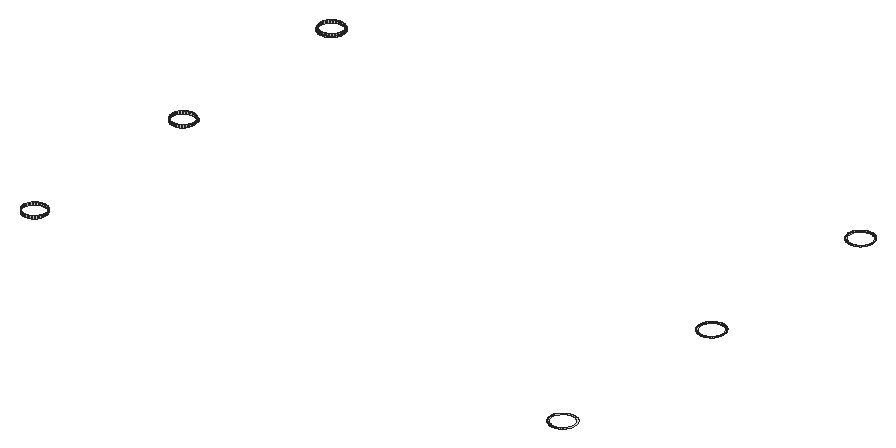
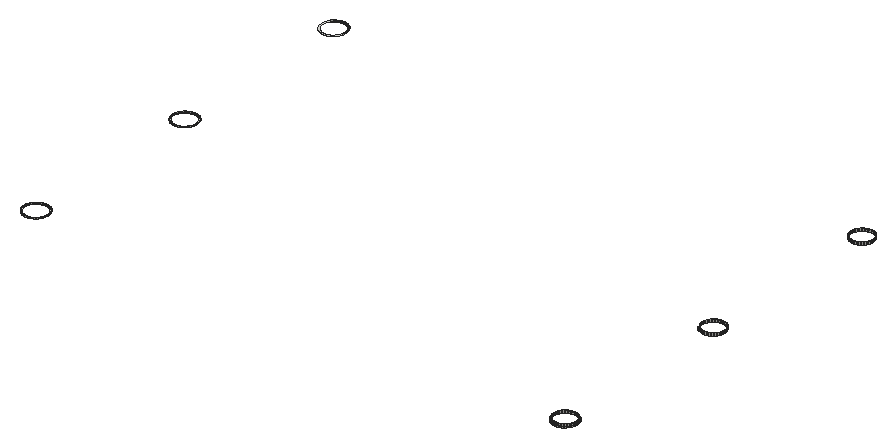
# SketchUp Ruby script. Lengths in inches.
U = 1.inch
M = Sketchup.active_model
def pt(a) = Geom::Point3d.new(a.map { |v| v * U })
def face(e, loops, mat)
  f = e.add_face(loops[0].map { |a| pt(a) })
  loops[1..].each { |l| e.add_face(l.map { |a| pt(a) }).erase! }
  f.material = f.back_material = mat if mat
  f
end
# faces: each face lists its corners as indices into pts; further lists are holes
def faces(e, pts, list, mat = nil) = list.each { |f| face(e, (f[0].is_a?(Array) ? f : [f]).map { |l| l.map { |i| pts[i] } }, mat) }
# xy, xz, yz: faces in a plane at the given z, y or x. An outline is a flat list of corners, or four numbers for a rectangle; further outlines are holes
def ring(l) = l.size == 4 ? [[l[0], l[1]], [l[2], l[1]], [l[2], l[3]], [l[0], l[3]]] : l.each_slice(2).to_a
def flat(e, list, mat, &to3) = list.each { |f| face(e, (f[0].is_a?(Array) ? f : [f]).map { |l| ring(l).map { |u, v| to3.(u, v) } }, mat) }
def xy(e, z, list, mat = nil) = flat(e, list, mat) { |x, y| [x, y, z] }
def xz(e, y, list, mat = nil) = flat(e, list, mat) { |x, z| [x, y, z] }
def yz(e, x, list, mat = nil) = flat(e, list, mat) { |y, z| [x, y, z] }
def lines(e, pts, list) = list.each { |a, b| e.add_line(pt(pts[a]), pt(pts[b])) }
# prism: a flat outline (further loops are holes) pulled along v
def prism(e, loops, v, mat = nil)
  f = face(e, loops, mat); d = Geom::Vector3d.new(v.map { |x| x * U })
  f.pushpull(f.normal.samedirection?(d) ? d.length : -d.length)
end
def box(e, o, s, mat = nil) = prism(e, [[o, [o[0] + s[0], o[1], o[2]], [o[0] + s[0], o[1] + s[1], o[2]], [o[0], o[1] + s[1], o[2]]]], [0, 0, s[2]], mat)
def at(x, y, z, deg = 0) = Geom::Transformation.translation(pt([x, y, z])) * Geom::Transformation.rotation(ORIGIN, Z_AXIS, deg.degrees)
def axes(o, x, y, z) = Geom::Transformation.new([*x, 0, *y, 0, *z, 0, *pt(o).to_a, 1])
def part(name) = M.definitions.add(name)
# library, detail: a bought-in or finely detailed component or shape, given as its bounding box
def library(name, o, s) = part(name).tap { |d| box(d.entities, o, s) }
def detail(e, o, s) = box(e.add_group.entities, o, s)
def put(e, d, t, mat = nil) = e.add_instance(d, t).tap { |i| i.material = mat if mat }
def group(e, t, mat = nil) = e.add_group.tap { |g| g.transformation = t; g.material = mat if mat }.entities
root = M.entities
xy(root,113.9,[[[112.03,39.21,111.8,39.22,111.57,39.26,111.35,39.3125,111.13,39.39,110.92,39.5,110.73,39.62,110.55,39.76,110.38,39.92,110.24,40.1,110.11,40.29,110,40.49,109.92,40.71,109.85,40.93,109.82,41.16,109.8,41.39,109.81,41.62,109.84,41.85,109.9,42.07,109.98,42.28,110.08,42.49,110.2,42.69,110.35,42.87,110.51,43.03,110.69,43.18,110.875,43.31,111.08,43.41,111.29,43.5,111.52,43.56,111.74,43.6,111.97,43.61,112.2,43.6,112.43,43.57,112.65,43.51,112.87,43.43,113.08,43.33,113.27,43.21,113.45,43.07,113.62,42.91,113.76,42.73,113.89,42.54,114,42.33,114.08,42.12,114.15,41.9,114.18,41.67,114.2,41.44,114.19,41.21,114.16,40.98,114.1,40.76,114.02,40.54,113.92,40.34,113.8,40.14,113.65,39.96,113.49,39.8,113.31,39.65,113.125,39.52,112.92,39.42,112.71,39.33,112.48,39.27,112.26,39.23],[112.02,39.41,112.23,39.43,112.44,39.46,112.64,39.52,112.84,39.6,113.02,39.69,113.2,39.8125,113.36,39.94,113.5,40.09,113.63,40.26,113.74,40.44,113.84,40.625,113.91,40.82,113.96,41.02,113.99,41.23,114,41.4375,113.99,41.65,113.95,41.85,113.89,42.06,113.82,42.25,113.72,42.44,113.6,42.61,113.47,42.77,113.32,42.92,113.16,43.05,112.98,43.16,112.79,43.25,112.59,43.32,112.39,43.375,112.18,43.41,111.98,43.41,111.77,43.4,111.56,43.37,111.36,43.31,111.16,43.23,110.98,43.13,110.8,43.02,110.64,42.88,110.5,42.73,110.37,42.57,110.26,42.39,110.16,42.21,110.09,42.01,110.04,41.81,110.01,41.6,110,41.39,110.01,41.18,110.05,40.97,110.11,40.77,110.18,40.58,110.28,40.39,110.4,40.22,110.53,40.06,110.68,39.91,110.84,39.78,111.02,39.67,111.21,39.58,111.41,39.5,111.61,39.45,111.82,39.42]],[[112.03,72.63,111.8,72.64,111.57,72.67,111.35,72.73,111.13,72.81,110.92,72.91,110.73,73.03,110.55,73.18,110.38,73.34,110.24,73.51,110.11,73.7,110,73.91,109.92,74.12,109.85,74.34,109.82,74.57,109.8,74.8,109.81,75.03,109.84,75.26,109.9,75.48,109.98,75.7,110.08,75.9,110.2,76.1,110.35,76.28,110.51,76.44,110.69,76.59,110.875,76.72,111.08,76.83,111.29,76.91,111.52,76.97,111.74,77.01,111.97,77.03,112.2,77.02,112.43,76.99,112.65,76.93,112.87,76.85,113.08,76.75,113.27,76.625,113.45,76.48,113.62,76.32,113.76,76.14,113.89,75.95,114,75.75,114.08,75.53,114.15,75.3125,114.18,75.08,114.2,74.86,114.19,74.625,114.16,74.4,114.1,74.17,114.02,73.96,113.92,73.75,113.8,73.56,113.65,73.375,113.49,73.21,113.31,73.0625,113.125,72.9375,112.92,72.83,112.71,72.74,112.48,72.68,112.26,72.64],[112.02,72.83,112.23,72.84,112.44,72.88,112.64,72.93,112.84,73.01,113.02,73.11,113.2,73.22,113.36,73.36,113.5,73.51,113.63,73.67,113.74,73.85,113.84,74.04,113.91,74.23,113.96,74.4375,113.99,74.64,114,74.85,113.99,75.0625,113.95,75.27,113.89,75.47,113.82,75.66,113.72,75.85,113.6,76.02,113.47,76.18,113.32,76.33,113.16,76.46,112.98,76.57,112.79,76.67,112.59,76.74,112.39,76.79,112.18,76.82,111.98,76.83,111.77,76.8125,111.56,76.78,111.36,76.72,111.16,76.65,110.98,76.55,110.8,76.43,110.64,76.3,110.5,76.15,110.37,75.98,110.26,75.81,110.16,75.62,110.09,75.42,110.04,75.22,110.01,75.01,110,74.8,110.01,74.59,110.05,74.39,110.11,74.1875,110.18,73.99,110.28,73.81,110.4,73.63,110.53,73.47,110.68,73.33,110.84,73.2,111.02,73.08,111.21,72.99,111.41,72.92,111.61,72.87,111.82,72.84]],[[112.03,106.04,111.8,106.05,111.57,106.08,111.35,106.14,111.13,106.22,110.92,106.32,110.73,106.45,110.55,106.59,110.38,106.75,110.24,106.93,110.11,107.12,110,107.32,109.92,107.54,109.85,107.76,109.82,107.99,109.8,108.22,109.81,108.45,109.84,108.67,109.9,108.9,109.98,109.11,110.08,109.32,110.2,109.51,110.35,109.69,110.51,109.86,110.69,110.01,110.875,110.13,111.08,110.24,111.29,110.33,111.52,110.39,111.74,110.43,111.97,110.44,112.2,110.43,112.43,110.4,112.65,110.34,112.87,110.26,113.08,110.16,113.27,110.04,113.45,109.9,113.62,109.73,113.76,109.56,113.89,109.37,114,109.16,114.08,108.95,114.15,108.73,114.18,108.5,114.2,108.27,114.19,108.04,114.16,107.8125,114.1,107.59,114.02,107.37,113.92,107.17,113.8,106.97,113.65,106.79,113.49,106.625,113.31,106.48,113.125,106.35,112.92,106.24,112.71,106.16,112.48,106.1,112.26,106.06],[112.02,106.24,112.23,106.26,112.44,106.29,112.64,106.35,112.84,106.43,113.02,106.52,113.2,106.64,113.36,106.77,113.5,106.92,113.63,107.09,113.74,107.26,113.84,107.45,113.91,107.65,113.96,107.85,113.99,108.06,114,108.27,113.99,108.48,113.95,108.68,113.89,108.88,113.82,109.08,113.72,109.26,113.6,109.4375,113.47,109.6,113.32,109.74,113.16,109.875,112.98,109.99,112.79,110.08,112.59,110.15,112.39,110.2,112.18,110.23,111.98,110.24,111.77,110.23,111.56,110.19,111.36,110.14,111.16,110.06,110.98,109.96,110.8,109.85,110.64,109.71,110.5,109.5625,110.37,109.4,110.26,109.22,110.16,109.03,110.09,108.84,110.04,108.63,110.01,108.43,110,108.22,110.01,108.01,110.05,107.8,110.11,107.6,110.18,107.41,110.28,107.22,110.4,107.05,110.53,106.89,110.68,106.74,110.84,106.61,111.02,106.5,111.21,106.41,111.41,106.33,111.61,106.28,111.82,106.25]],[[16.81,106.41,16.58,106.42,16.35,106.44,16.125,106.49,15.91,106.5625,15.7,106.66,15.5,106.77,15.31,106.91,15.14,107.0625,14.99,107.23,14.86,107.42,14.74,107.62,14.65,107.83,14.58,108.05,14.54,108.27,14.51,108.5,14.52,108.73,14.54,108.96,14.59,109.18,14.66,109.4,14.76,109.61,14.87,109.81,15.01,109.99,15.16,110.16,15.33,110.32,15.52,110.45,15.72,110.5625,15.93,110.66,16.15,110.73,16.375,110.77,16.6,110.8,16.83,110.79,17.06,110.77,17.28,110.72,17.5,110.65,17.71,110.55,17.91,110.4375,18.09,110.3,18.26,110.15,18.42,109.97,18.55,109.79,18.66,109.59,18.76,109.38,18.83,109.16,18.87,108.94,18.89,108.71,18.89,108.48,18.87,108.25,18.82,108.02,18.75,107.81,18.65,107.6,18.54,107.4,18.4,107.21,18.25,107.05,18.07,106.89,17.89,106.76,17.6875,106.65,17.48,106.55,17.26,106.48,17.03,106.4375],[16.8,106.61,17,106.63,17.21,106.68,17.41,106.74,17.6,106.82,17.78,106.93,17.95,107.05,18.11,107.1875,18.25,107.34,18.37,107.51,18.47,107.69,18.5625,107.88,18.625,108.08,18.67,108.28,18.69,108.49,18.7,108.7,18.67,108.9,18.63,109.11,18.57,109.31,18.49,109.5,18.38,109.68,18.26,109.85,18.12,110.01,17.97,110.15,17.8,110.27,17.62,110.375,17.43,110.46,17.23,110.53,17.03,110.57,16.82,110.59,16.61,110.6,16.4,110.57,16.2,110.53,16,110.47,15.81,110.39,15.63,110.28,15.46,110.16,15.3,110.02,15.16,109.87,15.04,109.7,14.93,109.52,14.85,109.33,14.78,109.13,14.74,108.93,14.72,108.72,14.71,108.51,14.73,108.3,14.78,108.1,14.84,107.9,14.92,107.71,15.03,107.53,15.15,107.36,15.29,107.2,15.44,107.0625,15.61,106.94,15.79,106.83,15.98,106.75,16.18,106.68,16.38,106.64,16.59,106.62]]])
xz(root,39.92,[[16.59,113.9,16.8,114.33]])
xz(root,43.9,[[16.61,113.9,16.82,114.33]])
xz(root,73.27,[[16.59,113.9,16.8,114.34]])
xz(root,77.25,[[16.61,113.9,16.82,114.34]])
yz(root,18.89,[[108.48,113.9,108.71,114]])
p = [[111.8,39.22,114],[111.57,39.26,114],[111.57,39.26,113.9],[111.8,39.22,113.9],[112.03,39.21,114],[112.03,39.21,113.9],
  [112.26,39.23,114],[112.26,39.23,113.9],[112.48,39.27,114],[112.48,39.27,113.9],[111.35,39.3125,114],[111.13,39.39,114],
  [111.13,39.39,113.9],[111.35,39.3125,113.9],[112.71,39.33,114],[112.71,39.33,113.9],[112.92,39.42,114],[112.92,39.42,113.9],
  [110.92,39.5,114],[110.92,39.5,113.9],[113.125,39.52,114],[113.125,39.52,113.9],[110.73,39.62,114],[110.73,39.62,113.9],
  [113.31,39.65,114],[113.31,39.65,113.9],[110.55,39.76,114],[110.55,39.76,113.9],[113.49,39.8,114],[113.49,39.8,113.9],
  [110.38,39.92,114],[110.38,39.92,113.9],[113.65,39.96,114],[113.65,39.96,113.9],[16.38,39.94,113.9],[16.18,39.99,113.9],
  [16.18,39.99,114.33],[16.38,39.94,114.33],[16.59,39.92,113.9],[16.59,39.92,114.33],[17,39.94,113.9],[16.8,39.92,113.9],
  [16.8,39.92,114.33],[17,39.94,114.33],[17.21,39.98,113.9],[17.21,39.98,114.33],[110.24,40.1,114],[110.24,40.1,113.9],
  [15.98,40.05,113.9],[15.98,40.05,114.33],[17.41,40.05,113.9],[17.41,40.05,114.33],[17.6,40.13,113.9],[17.6,40.13,114.33],
  [15.79,40.14,113.9],[15.61,40.25,113.9],[15.61,40.25,114.33],[15.79,40.14,114.33],[17.78,40.23,113.9],[17.78,40.23,114.33],
  [110.11,40.29,114],[110.11,40.29,113.9],[15.44,40.37,113.9],[15.44,40.37,114.33],[17.95,40.35,113.9],[17.95,40.35,114.33],
  [110,40.49,114],[110,40.49,113.9],[15.29,40.51,113.9],[15.29,40.51,114.33],[18.11,40.49,113.9],[18.11,40.49,114.33],
  [15.15,40.67,113.9],[15.15,40.67,114.33],[18.25,40.65,113.9],[18.25,40.65,114.33],[109.92,40.71,114],[109.92,40.71,113.9],
  [18.37,40.82,113.9],[18.37,40.82,114.33],[15.03,40.84,113.9],[15.03,40.84,114.33],[109.85,40.93,114],[109.85,40.93,113.9],
  [14.92,41.02,113.9],[14.92,41.02,114.33],[18.47,41,113.9],[18.47,41,114.33],[109.82,41.16,114],[109.82,41.16,113.9],
  [14.84,41.21,113.9],[14.84,41.21,114.33],[18.5625,41.1875,113.9],[18.5625,41.1875,114.33],[14.78,41.41,113.9],[14.78,41.41,114.33],
  [18.625,41.38,113.9],[18.625,41.38,114.33],[109.8,41.39,114],[109.8,41.39,113.9],[14.73,41.61,113.9],[14.73,41.61,114.33],
  [18.67,41.59,113.9],[18.67,41.59,114.33],[109.81,41.62,114],[109.81,41.62,113.9],[14.71,41.82,113.9],[14.71,41.82,114.33],
  [18.69,41.79,113.9],[18.69,41.79,114.33],[109.84,41.85,114],[109.84,41.85,113.9],[14.72,42.03,113.9],[14.72,42.03,114.33],
  [18.7,42,113.9],[18.7,42,114.33],[109.9,42.07,114],[109.9,42.07,113.9],[14.74,42.23,113.9],[14.74,42.23,114.33],
  [18.67,42.21,113.9],[18.67,42.21,114.33],[14.78,42.4375,113.9],[14.78,42.4375,114.33],[18.63,42.42,113.9],[18.63,42.42,114.33],
  [14.85,42.64,113.9],[14.85,42.64,114.33],[18.57,42.61,113.9],[18.57,42.61,114.33],[14.93,42.83,113.9],[14.93,42.83,114.33],
  [18.49,42.81,113.9],[18.49,42.81,114.33],[15.04,43.01,113.9],[15.04,43.01,114.33],[18.38,42.99,113.9],[18.38,42.99,114.33],
  [15.16,43.17,113.9],[15.16,43.17,114.33],[18.26,43.16,113.9],[18.26,43.16,114.33],[15.3,43.33,113.9],[15.3,43.33,114.33],
  [18.12,43.3125,113.9],[18.12,43.3125,114.33],[15.46,43.47,113.9],[15.46,43.47,114.33],[17.97,43.45,113.9],[17.97,43.45,114.33],
  [15.63,43.59,113.9],[15.63,43.59,114.33],[17.8,43.58,113.9],[17.8,43.58,114.33],[15.81,43.69,113.9],[15.81,43.69,114.33],
  [17.62,43.68,113.9],[17.62,43.68,114.33],[16,43.78,113.9],[16,43.78,114.33],[17.43,43.77,113.9],[17.43,43.77,114.33],
  [16.2,43.84,113.9],[16.2,43.84,114.33],[16.4,43.88,113.9],[16.4,43.88,114.33],[17.03,43.88,113.9],[17.23,43.83,113.9],
  [17.23,43.83,114.33],[17.03,43.88,114.33],[16.61,43.9,113.9],[16.61,43.9,114.33],[16.82,43.9,113.9],[16.82,43.9,114.33],
  [111.8,72.64,114],[111.57,72.67,114],[111.57,72.67,113.9],[111.8,72.64,113.9],[112.03,72.63,114],[112.03,72.63,113.9],
  [112.26,72.64,114],[112.26,72.64,113.9],[112.48,72.68,114],[112.48,72.68,113.9],[111.35,72.73,114],[111.13,72.81,114],
  [111.13,72.81,113.9],[111.35,72.73,113.9],[112.71,72.74,114],[112.71,72.74,113.9],[112.92,72.83,114],[112.92,72.83,113.9],
  [110.92,72.91,114],[110.92,72.91,113.9],[113.125,72.9375,114],[113.125,72.9375,113.9],[110.73,73.03,114],[110.73,73.03,113.9],
  [113.31,73.0625,114],[113.31,73.0625,113.9],[110.55,73.18,114],[110.55,73.18,113.9],[113.49,73.21,114],[113.49,73.21,113.9],
  [110.38,73.34,114],[110.38,73.34,113.9],[113.65,73.375,114],[113.65,73.375,113.9],[16.18,73.34,113.9],[15.98,73.4,113.9],
  [15.98,73.4,114.34],[16.18,73.34,114.34],[16.38,73.29,113.9],[16.38,73.29,114.34],[16.59,73.27,113.9],[16.59,73.27,114.34],
  [17,73.29,113.9],[16.8,73.27,113.9],[16.8,73.27,114.34],[17,73.29,114.34],[17.21,73.33,113.9],[17.21,73.33,114.34],
  [17.41,73.39,113.9],[17.41,73.39,114.34],[110.24,73.51,114],[110.24,73.51,113.9],[15.79,73.49,113.9],[15.79,73.49,114.34],
  [17.6,73.48,113.9],[17.6,73.48,114.34],[113.8,73.56,114],[113.8,73.56,113.9],[15.61,73.59,113.9],[15.61,73.59,114.34],
  [17.78,73.58,113.9],[17.78,73.58,114.34],[110.11,73.7,114],[110.11,73.7,113.9],[15.44,73.72,113.9],[15.44,73.72,114.34],
  [17.95,73.7,113.9],[17.95,73.7,114.34],[113.92,73.75,114],[113.92,73.75,113.9],[15.29,73.86,113.9],[15.29,73.86,114.34],
  [18.11,73.84,113.9],[18.11,73.84,114.34],[110,73.91,114],[110,73.91,113.9],[18.25,73.99,113.9],[18.25,73.99,114.34],
  [114.02,73.96,114],[114.02,73.96,113.9],[15.15,74.01,113.9],[15.15,74.01,114.34],[109.92,74.12,114],[109.92,74.12,113.9],
  [15.03,74.18,113.9],[15.03,74.18,114.34],[18.37,74.16,113.9],[18.37,74.16,114.34],[114.1,74.17,114],[114.1,74.17,113.9],
  [109.85,74.34,114],[109.85,74.34,113.9],[14.92,74.36,113.9],[14.92,74.36,114.34],[18.47,74.34,113.9],[18.47,74.34,114.34],
  [114.16,74.4,114],[114.16,74.4,113.9],[18.5625,74.53,113.9],[18.5625,74.53,114.34],[109.82,74.57,114],[109.82,74.57,113.9],
  [14.84,74.55,113.9],[14.84,74.55,114.34],[114.19,74.625,114],[114.19,74.625,113.9],[18.625,74.73,113.9],[18.625,74.73,114.34],
  [14.78,74.75,113.9],[14.78,74.75,114.34],[109.8,74.8,114],[109.8,74.8,113.9],[114.2,74.86,114],[114.2,74.86,113.9],
  [18.67,74.93,113.9],[18.67,74.93,114.34],[14.73,74.96,113.9],[14.73,74.96,114.34],[109.81,75.03,114],[109.81,75.03,113.9],
  [18.69,75.14,113.9],[18.69,75.14,114.34],[114.18,75.08,114],[114.18,75.08,113.9],[14.71,75.17,113.9],[14.71,75.17,114.34],
  [109.84,75.26,114],[109.84,75.26,113.9],[18.7,75.35,113.9],[18.7,75.35,114.34],[114.15,75.3125,114],[114.15,75.3125,113.9],
  [14.72,75.375,113.9],[14.72,75.375,114.34],[109.9,75.48,114],[109.9,75.48,113.9],[114.08,75.53,114],[114.08,75.53,113.9],
  [14.74,75.58,113.9],[14.74,75.58,114.34],[18.67,75.56,113.9],[18.67,75.56,114.34],[109.98,75.7,114],[109.98,75.7,113.9],
  [114,75.75,114],[114,75.75,113.9],[14.78,75.78,113.9],[14.78,75.78,114.34],[18.63,75.76,113.9],[18.63,75.76,114.34],
  [110.08,75.9,114],[110.08,75.9,113.9],[113.89,75.95,114],[113.89,75.95,113.9],[14.85,75.98,113.9],[14.85,75.98,114.34],
  [18.57,75.96,113.9],[18.57,75.96,114.34],[110.2,76.1,114],[110.2,76.1,113.9],[14.93,76.17,113.9],[14.93,76.17,114.34],
  [18.49,76.15,113.9],[18.49,76.15,114.34],[113.76,76.14,114],[113.76,76.14,113.9],[110.35,76.28,114],[110.35,76.28,113.9],
  [113.62,76.32,114],[113.62,76.32,113.9],[15.04,76.35,113.9],[15.04,76.35,114.34],[18.38,76.33,113.9],[18.38,76.33,114.34],
  [18.55,76.44,114],[18.66,76.24,114],[18.66,76.24,113.9],[18.55,76.44,113.9],[18.26,76.5,113.9],[18.26,76.5,114.34],
  [110.51,76.44,114],[110.51,76.44,113.9],[113.45,76.48,114],[113.45,76.48,113.9],[15.16,76.52,113.9],[15.16,76.52,114.34],
  [18.42,76.63,114],[18.42,76.63,113.9],[110.69,76.59,114],[110.69,76.59,113.9],[15.3,76.68,113.9],[15.3,76.68,114.34],
  [18.12,76.66,113.9],[18.12,76.66,114.34],[113.27,76.625,114],[113.27,76.625,113.9],[18.26,76.8,114],[18.26,76.8,113.9],
  [110.875,76.72,114],[110.875,76.72,113.9],[113.08,76.75,114],[113.08,76.75,113.9],[15.46,76.8125,113.9],[15.46,76.8125,114.34],
  [17.97,76.8,113.9],[17.97,76.8,114.34],[111.08,76.83,114],[111.08,76.83,113.9],[112.87,76.85,114],[112.87,76.85,113.9],
  [15.63,76.9375,113.9],[15.63,76.9375,114.34],[17.8,76.92,113.9],[17.8,76.92,114.34],[18.09,76.95,114],[18.09,76.95,113.9],
  [111.29,76.91,114],[111.29,76.91,113.9],[112.65,76.93,114],[112.65,76.93,113.9],[15.81,77.04,113.9],[15.81,77.04,114.34],
  [17.62,77.03,113.9],[17.62,77.03,114.34],[111.52,76.97,114],[111.52,76.97,113.9],[112.43,76.99,114],[112.43,76.99,113.9],
  [16,77.12,113.9],[16,77.12,114.34],[17.43,77.11,113.9],[17.43,77.11,114.34],[17.91,77.09,114],[17.91,77.09,113.9],
  [111.74,77.01,114],[111.74,77.01,113.9],[111.97,77.03,114],[111.97,77.03,113.9],[112.2,77.02,114],[112.2,77.02,113.9],
  [16.2,77.1875,113.9],[16.2,77.1875,114.34],[17.23,77.18,113.9],[17.23,77.18,114.34],[16.4,77.23,113.9],[16.4,77.23,114.34],
  [16.61,77.25,113.9],[16.61,77.25,114.34],[16.82,77.25,113.9],[17.03,77.22,113.9],[17.03,77.22,114.34],[16.82,77.25,114.34],
  [112.03,106.04,114],[111.8,106.05,114],[111.8,106.05,113.9],[112.03,106.04,113.9],[112.26,106.06,114],[112.26,106.06,113.9],
  [111.35,106.14,114],[111.13,106.22,114],[111.13,106.22,113.9],[111.35,106.14,113.9],[111.57,106.08,114],[111.57,106.08,113.9],
  [112.48,106.1,114],[112.48,106.1,113.9],[112.71,106.16,114],[112.71,106.16,113.9],[110.92,106.32,114],[110.92,106.32,113.9],
  [112.92,106.24,114],[112.92,106.24,113.9],[113.125,106.35,114],[113.125,106.35,113.9],[110.73,106.45,114],[110.73,106.45,113.9],
  [16.35,106.44,114],[16.125,106.49,114],[16.125,106.49,113.9],[16.35,106.44,113.9],[16.58,106.42,114],[16.58,106.42,113.9],
  [16.81,106.41,114],[16.81,106.41,113.9],[17.03,106.4375,114],[17.03,106.4375,113.9],[17.26,106.48,114],[17.26,106.48,113.9],
  [110.55,106.59,114],[110.55,106.59,113.9],[113.31,106.48,114],[113.31,106.48,113.9],[15.91,106.5625,114],[15.91,106.5625,113.9],
  [17.48,106.55,114],[17.48,106.55,113.9],[113.49,106.625,114],[113.49,106.625,113.9],[15.7,106.66,114],[15.7,106.66,113.9],
  [16.38,106.64,113.9],[16.18,106.68,113.9],[16.18,106.68,114.34],[16.38,106.64,114.34],[16.59,106.62,113.9],[16.59,106.62,114.34],
  [16.8,106.61,113.9],[16.8,106.61,114.34],[17,106.63,113.9],[17,106.63,114.34],[17.21,106.68,113.9],[17.21,106.68,114.34],
  [17.6875,106.65,114],[17.6875,106.65,113.9],[17.89,106.76,114],[17.89,106.76,113.9],[110.38,106.75,114],[110.38,106.75,113.9],
  [113.65,106.79,114],[113.65,106.79,113.9],[15.5,106.77,114],[15.5,106.77,113.9],[15.98,106.75,113.9],[15.79,106.83,113.9],
  [15.79,106.83,114.34],[15.98,106.75,114.34],[17.41,106.74,113.9],[17.41,106.74,114.34],[17.6,106.82,113.9],[17.6,106.82,114.34],
  [15.31,106.91,114],[15.31,106.91,113.9],[15.61,106.94,113.9],[15.61,106.94,114.34],[17.78,106.93,113.9],[17.78,106.93,114.34],
  [18.07,106.89,114],[18.07,106.89,113.9],[110.24,106.93,114],[110.24,106.93,113.9],[113.8,106.97,114],[113.8,106.97,113.9],
  [15.14,107.0625,114],[15.14,107.0625,113.9],[15.44,107.0625,113.9],[15.44,107.0625,114.34],[17.95,107.05,113.9],[17.95,107.05,114.34],
  [18.25,107.05,114],[18.25,107.05,113.9],[110.11,107.12,114],[110.11,107.12,113.9],[18.11,107.1875,113.9],[18.11,107.1875,114.34],
  [18.4,107.21,114],[18.4,107.21,113.9],[113.92,107.17,114],[113.92,107.17,113.9],[14.99,107.23,114],[14.99,107.23,113.9],
  [15.29,107.2,113.9],[15.29,107.2,114.34],[110,107.32,114],[110,107.32,113.9],[14.86,107.42,114],[14.86,107.42,113.9],
  [15.15,107.36,113.9],[15.15,107.36,114.34],[18.25,107.34,113.9],[18.25,107.34,114.34],[18.54,107.4,114],[18.54,107.4,113.9],
  [114.02,107.37,114],[114.02,107.37,113.9],[18.37,107.51,113.9],[18.37,107.51,114.34],[109.92,107.54,114],[109.92,107.54,113.9],
  [14.74,107.62,114],[14.74,107.62,113.9],[15.03,107.53,113.9],[15.03,107.53,114.34],[18.65,107.6,114],[18.65,107.6,113.9],
  [114.1,107.59,114],[114.1,107.59,113.9],[14.92,107.71,113.9],[14.92,107.71,114.34],[18.47,107.69,113.9],[18.47,107.69,114.34],
  [109.85,107.76,114],[109.85,107.76,113.9],[14.65,107.83,114],[14.65,107.83,113.9],[18.75,107.81,114],[18.75,107.81,113.9],
  [114.16,107.8125,114],[114.16,107.8125,113.9],[14.84,107.9,113.9],[14.84,107.9,114.34],[18.5625,107.88,113.9],[18.5625,107.88,114.34],
  [14.58,108.05,114],[14.58,108.05,113.9],[18.82,108.02,114],[18.82,108.02,113.9],[109.82,107.99,114],[109.82,107.99,113.9],
  [114.19,108.04,114],[114.19,108.04,113.9],[14.78,108.1,113.9],[14.78,108.1,114.34],[18.625,108.08,113.9],[18.625,108.08,114.34],
  [14.54,108.27,114],[14.54,108.27,113.9],[18.87,108.25,114],[18.87,108.25,113.9],[109.8,108.22,114],[109.8,108.22,113.9],
  [114.2,108.27,114],[114.2,108.27,113.9],[14.73,108.3,113.9],[14.73,108.3,114.34],[18.67,108.28,113.9],[18.67,108.28,114.34],
  [18.89,108.48,114],[18.89,108.48,113.9],[109.81,108.45,114],[109.81,108.45,113.9],[14.51,108.5,114],[14.51,108.5,113.9],
  [14.71,108.51,113.9],[14.71,108.51,114.34],[18.69,108.49,113.9],[18.69,108.49,114.34],[114.18,108.5,114],[114.18,108.5,113.9],
  [109.84,108.67,114],[109.84,108.67,113.9],[14.52,108.73,114],[14.52,108.73,113.9],[14.72,108.72,113.9],[14.72,108.72,114.34],
  [18.7,108.7,113.9],[18.7,108.7,114.34],[114.15,108.73,114],[114.15,108.73,113.9],[14.54,108.96,114],[14.54,108.96,113.9],
  [14.74,108.93,113.9],[14.74,108.93,114.34],[18.67,108.9,113.9],[18.67,108.9,114.34],[18.87,108.94,114],[18.89,108.71,114],
  [18.89,108.71,113.9],[18.87,108.94,113.9],[109.9,108.9,114],[109.9,108.9,113.9],[114.08,108.95,114],[114.08,108.95,113.9],
  [14.78,109.13,113.9],[14.78,109.13,114.34],[18.63,109.11,113.9],[18.63,109.11,114.34],[18.83,109.16,114],[18.83,109.16,113.9],
  [109.98,109.11,114],[109.98,109.11,113.9],[114,109.16,114],[114,109.16,113.9],[14.59,109.18,114],[14.59,109.18,113.9],
  [14.85,109.33,113.9],[14.85,109.33,114.34],[18.57,109.31,113.9],[18.57,109.31,114.34],[110.08,109.32,114],[110.08,109.32,113.9],
  [14.66,109.4,114],[14.66,109.4,113.9],[18.76,109.38,114],[18.76,109.38,113.9],[113.89,109.37,114],[113.89,109.37,113.9],
  [14.93,109.52,113.9],[14.93,109.52,114.34],[18.49,109.5,113.9],[18.49,109.5,114.34],[110.2,109.51,114],[110.2,109.51,113.9],
  [14.76,109.61,114],[14.76,109.61,113.9],[18.66,109.59,114],[18.66,109.59,113.9],[113.76,109.56,114],[113.76,109.56,113.9],
  [15.04,109.7,113.9],[15.04,109.7,114.34],[18.38,109.68,113.9],[18.38,109.68,114.34],[110.35,109.69,114],[110.35,109.69,113.9],
  [14.87,109.81,114],[14.87,109.81,113.9],[18.55,109.79,114],[18.55,109.79,113.9],[113.62,109.73,114],[113.62,109.73,113.9],
  [15.16,109.87,113.9],[15.16,109.87,114.34],[18.26,109.85,113.9],[18.26,109.85,114.34],[110.51,109.86,114],[110.51,109.86,113.9],
  [113.45,109.9,114],[113.45,109.9,113.9],[15.01,109.99,114],[15.01,109.99,113.9],[18.12,110.01,113.9],[18.12,110.01,114.34],
  [18.42,109.97,114],[18.42,109.97,113.9],[15.3,110.02,113.9],[15.3,110.02,114.34],[110.69,110.01,114],[110.69,110.01,113.9],
  [113.27,110.04,114],[113.27,110.04,113.9],[15.16,110.16,114],[15.16,110.16,113.9],[15.46,110.16,113.9],[15.46,110.16,114.34],
  [17.97,110.15,113.9],[17.97,110.15,114.34],[18.26,110.15,114],[18.26,110.15,113.9],[110.875,110.13,114],[110.875,110.13,113.9],
  [113.08,110.16,114],[113.08,110.16,113.9],[17.8,110.27,113.9],[17.8,110.27,114.34],[18.09,110.3,114],[18.09,110.3,113.9],
  [111.08,110.24,114],[111.08,110.24,113.9],[15.33,110.32,114],[15.33,110.32,113.9],[15.63,110.28,113.9],[15.63,110.28,114.34],
  [111.29,110.33,114],[111.29,110.33,113.9],[112.87,110.26,114],[112.87,110.26,113.9],[15.52,110.45,114],[15.52,110.45,113.9],
  [15.81,110.39,113.9],[15.81,110.39,114.34],[17.62,110.375,113.9],[17.62,110.375,114.34],[17.91,110.4375,114],[17.91,110.4375,113.9],
  [111.52,110.39,114],[111.52,110.39,113.9],[112.43,110.4,114],[112.65,110.34,114],[112.65,110.34,113.9],[112.43,110.4,113.9],
  [16,110.47,113.9],[16,110.47,114.34],[17.43,110.46,113.9],[17.43,110.46,114.34],[17.71,110.55,114],[17.71,110.55,113.9],
  [111.74,110.43,114],[111.74,110.43,113.9],[111.97,110.44,114],[111.97,110.44,113.9],[112.2,110.43,114],[112.2,110.43,113.9],
  [15.72,110.5625,114],[15.72,110.5625,113.9],[16.2,110.53,113.9],[16.2,110.53,114.34],[16.4,110.57,113.9],[16.4,110.57,114.34],
  [17.03,110.57,113.9],[17.23,110.53,113.9],[17.23,110.53,114.34],[17.03,110.57,114.34],[15.93,110.66,114],[15.93,110.66,113.9],
  [16.61,110.6,113.9],[16.61,110.6,114.34],[16.82,110.59,113.9],[16.82,110.59,114.34],[17.28,110.72,114],[17.5,110.65,114],
  [17.5,110.65,113.9],[17.28,110.72,113.9],[16.15,110.73,114],[16.15,110.73,113.9],[16.375,110.77,114],[16.375,110.77,113.9],
  [17.06,110.77,114],[17.06,110.77,113.9],[16.6,110.8,114],[16.6,110.8,113.9],[16.83,110.79,114],[16.83,110.79,113.9]]
faces(root,p,[[0,1,2,3],[4,0,3,5],[6,4,5,7],[8,6,7,9],[10,11,12,13],[1,10,13,2],[14,8,9,15],[16,14,15,17],
  [11,18,19,12],[20,16,17,21],[18,22,23,19],[24,20,21,25],[22,26,27,23],[28,24,25,29],[26,30,31,27],[32,28,29,33],
  [34,35,36,37],[38,34,37,39],[40,41,42,43],[44,40,43,45],[30,46,47,31],[35,48,49,36],[50,44,45,51],[52,50,51,53],
  [54,55,56,57],[48,54,57,49],[58,52,53,59],[46,60,61,47],[55,62,63,56],[64,58,59,65],[60,66,67,61],[62,68,69,63],
  [70,64,65,71],[68,72,73,69],[74,70,71,75],[66,76,77,67],[78,74,75,79],[72,80,81,73],[76,82,83,77],[80,84,85,81],
  [86,78,79,87],[82,88,89,83],[84,90,91,85],[92,86,87,93],[90,94,95,91],[96,92,93,97],[88,98,99,89],[94,100,101,95],
  [102,96,97,103],[98,104,105,99],[100,106,107,101],[108,102,103,109],[104,110,111,105],[106,112,113,107],[114,108,109,115],[110,116,117,111],
  [112,118,119,113],[120,114,115,121],[118,122,123,119],[124,120,121,125],[122,126,127,123],[128,124,125,129],[126,130,131,127],[132,128,129,133],
  [130,134,135,131],[136,132,133,137],[134,138,139,135],[140,136,137,141],[138,142,143,139],[144,140,141,145],[142,146,147,143],[148,144,145,149],
  [146,150,151,147],[152,148,149,153],[150,154,155,151],[156,152,153,157],[154,158,159,155],[160,156,157,161],[158,162,163,159],[162,164,165,163],
  [166,167,168,169],[167,160,161,168],[164,170,171,165],[172,166,169,173],[174,175,176,177],[178,174,177,179],[180,178,179,181],[182,180,181,183],
  [184,185,186,187],[175,184,187,176],[188,182,183,189],[190,188,189,191],[185,192,193,186],[194,190,191,195],[192,196,197,193],[198,194,195,199],
  [196,200,201,197],[202,198,199,203],[200,204,205,201],[206,202,203,207],[208,209,210,211],[212,208,211,213],[214,212,213,215],[216,217,218,219],
  [220,216,219,221],[222,220,221,223],[204,224,225,205],[209,226,227,210],[228,222,223,229],[230,206,207,231],[226,232,233,227],[234,228,229,235],
  [224,236,237,225],[232,238,239,233],[240,234,235,241],[242,230,231,243],[238,244,245,239],[246,240,241,247],[236,248,249,237],[250,246,247,251],
  [252,242,243,253],[244,254,255,245],[248,256,257,249],[254,258,259,255],[260,250,251,261],[262,252,253,263],[256,264,265,257],[258,266,267,259],
  [268,260,261,269],[270,262,263,271],[272,268,269,273],[264,274,275,265],[266,276,277,267],[278,270,271,279],[280,272,273,281],[276,282,283,277],
  [274,284,285,275],[286,278,279,287],[288,280,281,289],[282,290,291,283],[284,292,293,285],[294,288,289,295],[296,286,287,297],[290,298,299,291],
  [292,300,301,293],[302,294,295,303],[304,296,297,305],[298,306,307,299],[300,308,309,301],[310,304,305,311],[306,312,313,307],[314,302,303,315],
  [308,316,317,309],[318,310,311,319],[312,320,321,313],[322,314,315,323],[316,324,325,317],[326,318,319,327],[320,328,329,321],[330,322,323,331],
  [324,332,333,325],[328,334,335,329],[336,330,331,337],[338,326,327,339],[332,340,341,333],[342,338,339,343],[334,344,345,335],[346,336,337,347],
  [348,349,350,351],[352,346,347,353],[340,354,355,341],[356,342,343,357],[344,358,359,345],[360,348,351,361],[354,362,363,355],[358,364,365,359],
  [366,352,353,367],[368,356,357,369],[370,360,361,371],[362,372,373,363],[374,368,369,375],[364,376,377,365],[378,366,367,379],[372,380,381,373],
  [382,374,375,383],[376,384,385,377],[386,378,379,387],[388,370,371,389],[380,390,391,381],[392,382,383,393],[384,394,395,385],[396,386,387,397],
  [390,398,399,391],[400,392,393,401],[394,402,403,395],[404,396,397,405],[406,388,389,407],[398,408,409,399],[408,410,411,409],[410,412,413,411],
  [412,400,401,413],[402,414,415,403],[416,404,405,417],[414,418,419,415],[418,420,421,419],[422,423,424,425],[423,416,417,424],[426,427,428,429],
  [430,426,429,431],[432,433,434,435],[436,432,435,437],[427,436,437,428],[438,430,431,439],[440,438,439,441],[433,442,443,434],[444,440,441,445],
  [446,444,445,447],[442,448,449,443],[450,451,452,453],[454,450,453,455],[456,454,455,457],[458,456,457,459],[460,458,459,461],[448,462,463,449],
  [464,446,447,465],[451,466,467,452],[468,460,461,469],[470,464,465,471],[466,472,473,467],[474,475,476,477],[478,474,477,479],[480,478,479,481],
  [482,480,481,483],[484,482,483,485],[486,468,469,487],[488,486,487,489],[462,490,491,463],[492,470,471,493],[472,494,495,473],[496,497,498,499],
  [475,496,499,476],[500,484,485,501],[502,500,501,503],[494,504,505,495],[497,506,507,498],[508,502,503,509],[510,488,489,511],[490,512,513,491],
  [514,492,493,515],[504,516,517,505],[506,518,519,507],[520,508,509,521],[522,510,511,523],[512,524,525,513],[526,520,521,527],[528,522,523,529],
  [530,514,515,531],[516,532,533,517],[518,534,535,519],[524,536,537,525],[532,538,539,533],[534,540,541,535],[542,526,527,543],[544,528,529,545],
  [546,530,531,547],[548,542,543,549],[536,550,551,537],[538,552,553,539],[540,554,555,541],[556,544,545,557],[558,546,547,559],[554,560,561,555],
  [562,548,549,563],[550,564,565,551],[552,566,567,553],[568,556,557,569],[570,558,559,571],[560,572,573,561],[574,562,563,575],[566,576,577,567],
  [578,568,569,579],[564,580,581,565],[582,570,571,583],[572,584,585,573],[586,574,575,587],[576,588,589,577],[590,578,579,591],[580,592,593,581],
  [594,582,583,595],[584,596,597,585],[598,586,587,599],[600,590,591,601],[592,602,603,593],[588,604,605,589],[596,606,607,597],[608,598,599,609],
  [610,594,595,611],[602,612,613,603],[604,614,615,605],[606,616,617,607],[618,608,609,619],[620,610,611,621],[614,622,623,615],[616,624,625,617],
  [626,618,619,627],[628,629,630,631],[612,632,633,613],[634,620,621,635],[624,636,637,625],[638,626,627,639],[640,628,631,641],[632,642,643,633],
  [644,634,635,645],[622,646,647,623],[636,648,649,637],[650,638,639,651],[642,652,653,643],[646,654,655,647],[656,640,641,657],[658,644,645,659],
  [648,660,661,649],[662,650,651,663],[652,664,665,653],[654,666,667,655],[668,656,657,669],[670,658,659,671],[660,672,673,661],[674,662,663,675],
  [664,676,677,665],[666,678,679,667],[680,668,669,681],[682,670,671,683],[672,684,685,673],[686,674,675,687],[676,688,689,677],[690,682,683,691],
  [678,692,693,679],[694,686,687,695],[696,680,681,697],[684,698,699,685],[688,700,701,689],[702,690,691,703],[692,704,705,693],[698,706,707,699],
  [708,694,695,709],[710,696,697,711],[700,712,713,701],[714,702,703,715],[716,708,709,717],[718,710,711,719],[712,720,721,713],[704,722,723,705],
  [706,724,725,707],[720,726,727,721],[728,714,715,729],[722,730,731,723],[724,732,733,725],[734,716,717,735],[736,718,719,737],[726,738,739,727],
  [740,741,742,743],[741,728,729,742],[732,744,745,733],[746,734,735,747],[748,736,737,749],[738,750,751,739],[750,752,753,751],[752,754,755,753],
  [754,740,743,755],[730,756,757,731],[744,758,759,745],[758,760,761,759],[762,763,764,765],[763,746,747,764],[756,766,767,757],[760,768,769,761],
  [768,770,771,769],[770,762,765,771],[772,773,774,775],[773,748,749,774],[766,776,777,767],[776,778,779,777],[780,772,775,781],[778,782,783,779],
  [782,784,785,783],[784,780,781,785]])
